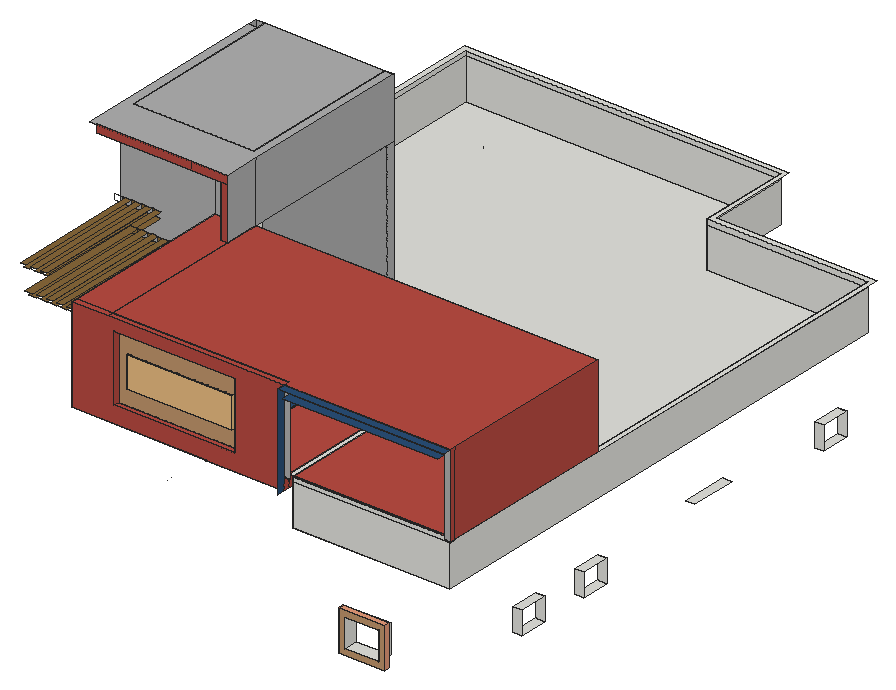
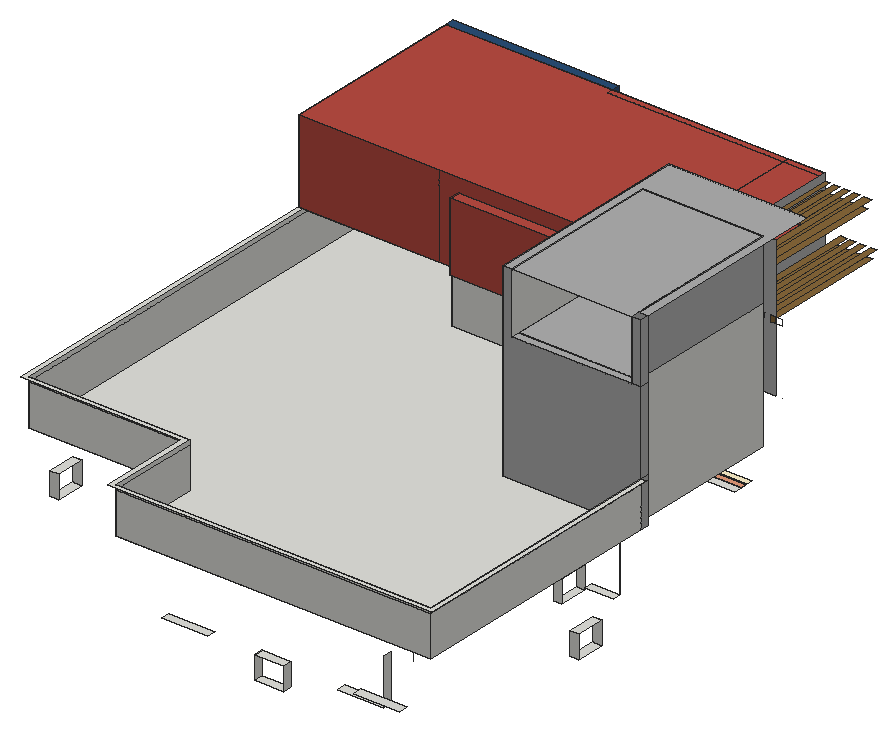
# SketchUp Ruby script. Lengths in inches.
U = 1.inch
M = Sketchup.active_model
def pt(a) = Geom::Point3d.new(a.map { |v| v * U })
def face(e, loops, mat)
  f = e.add_face(loops[0].map { |a| pt(a) })
  loops[1..].each { |l| e.add_face(l.map { |a| pt(a) }).erase! }
  f.material = f.back_material = mat if mat
  f
end
# faces: each face lists its corners as indices into pts; further lists are holes
def faces(e, pts, list, mat = nil) = list.each { |f| face(e, (f[0].is_a?(Array) ? f : [f]).map { |l| l.map { |i| pts[i] } }, mat) }
# xy, xz, yz: faces in a plane at the given z, y or x. An outline is a flat list of corners, or four numbers for a rectangle; further outlines are holes
def ring(l) = l.size == 4 ? [[l[0], l[1]], [l[2], l[1]], [l[2], l[3]], [l[0], l[3]]] : l.each_slice(2).to_a
def flat(e, list, mat, &to3) = list.each { |f| face(e, (f[0].is_a?(Array) ? f : [f]).map { |l| ring(l).map { |u, v| to3.(u, v) } }, mat) }
def xy(e, z, list, mat = nil) = flat(e, list, mat) { |x, y| [x, y, z] }
def xz(e, y, list, mat = nil) = flat(e, list, mat) { |x, z| [x, y, z] }
def yz(e, x, list, mat = nil) = flat(e, list, mat) { |y, z| [x, y, z] }
def lines(e, pts, list) = list.each { |a, b| e.add_line(pt(pts[a]), pt(pts[b])) }
# prism: a flat outline (further loops are holes) pulled along v
def prism(e, loops, v, mat = nil)
  f = face(e, loops, mat); d = Geom::Vector3d.new(v.map { |x| x * U })
  f.pushpull(f.normal.samedirection?(d) ? d.length : -d.length)
end
def box(e, o, s, mat = nil) = prism(e, [[o, [o[0] + s[0], o[1], o[2]], [o[0] + s[0], o[1] + s[1], o[2]], [o[0], o[1] + s[1], o[2]]]], [0, 0, s[2]], mat)
def at(x, y, z, deg = 0) = Geom::Transformation.translation(pt([x, y, z])) * Geom::Transformation.rotation(ORIGIN, Z_AXIS, deg.degrees)
def axes(o, x, y, z) = Geom::Transformation.new([*x, 0, *y, 0, *z, 0, *pt(o).to_a, 1])
def part(name) = M.definitions.add(name)
# library, detail: a bought-in or finely detailed component or shape, given as its bounding box
def library(name, o, s) = part(name).tap { |d| box(d.entities, o, s) }
def detail(e, o, s) = box(e.add_group.entities, o, s)
def put(e, d, t, mat = nil) = e.add_instance(d, t).tap { |i| i.material = mat if mat }
def group(e, t, mat = nil) = e.add_group.tap { |g| g.transformation = t; g.material = mat if mat }.entities
root = M.entities
M.materials.add("Heather_Jeans").color = [86, 117, 147]
M.materials.add("Heather_PantShadow").color = [42, 79, 119]
M.materials.add("Heather_Skin").color = [229, 155, 121]
M.materials.add("K359").color = [135, 104, 58]
M.materials.add("Material~76").color = [176, 176, 176]
M.materials.add("Material~8").color = [65, 47, 38]
M.materials.add("Panel-Opening1").color = [194, 151, 109]
M.materials.add("[Color_D05]").color = [255, 242, 204]
M.materials.add("[Metal Rusted]").color = [184, 75, 66]
M.materials.add("[Polished Concrete New]").color = [200, 200, 203]
c1 = library("Eshavasya",[1,0,0],[56.875,16.44,1])
xy(root,52.62,[[93.01,603.52,141.01,612.52]])
xy(root,54,[[398.62,2.875,446.62,8.875]],"Heather_Skin")
xy(root,60,[[404.62,2.875,440.62,17.875]])
xy(root,66,[[501.9,101.875,510.9,131.875],[501.9,182.875,510.9,212.875],[3.9,439.375,12.9,469.375],[501.9,496.375,510.9,526.375],[158.71,652.375,188.71,661.375]])
xy(root,76.62,[[60.01,390.52,69.01,420.52]])
xy(root,90,[[404.62,2.875,440.62,17.875],[501.9,101.875,510.9,131.875],[395.4,161.875,425.4,167.875],[501.9,182.875,510.9,212.875],[177.5,190.375,249.5,205.375],
  [51.9,196.375,99.9,205.375],[287.9,196.375,327.9,205.375],[501.9,327.95,510.9,375.95],[17.9,397.375,47.9,406.375],[110.9,397.375,150.9,406.375],
  [3.9,439.375,12.9,469.375],[342.9,451.375,399.9,460.375],[399.9,464.375,405.9,494.375],[501.9,496.375,510.9,526.375],[167.9,499.375,203.9,508.375],
  [217.9,499.375,253.9,508.375],[173.9,556.375,203.9,562.375],[36.9,652.375,84.9,661.375],[158.71,652.375,188.71,661.375],[237.9,652.375,285.9,661.375]])
xy(root,90,[[51.9,190.375,99.9,196.375]],"Heather_Skin")
xy(root,96,[[398.62,2.875,446.62,8.875]],"Heather_Skin")
xy(root,96.08,[[45.9,190.375,105.9,196.375]],"[Color_D05]")
xy(root,96.18,[[171.5,190.375,255.5,191.8125]],"Heather_PantShadow")
xy(root,96.18,[[216.0625,191.8125,255.5,196.375]],"[Metal Rusted]")
xy(root,100.62,[[60.01,390.52,69.01,420.52]])
xy(root,108.3125,[[165.5,191.8125,165.55,196.375]],"[Metal Rusted]")
xy(root,108.37,[[165.55,191.8125,171.5,196.375]],"[Metal Rusted]")
xy(root,116.53,[[150.06,191.8125,150.19,196.375]],"[Metal Rusted]")
xy(root,146.6875,[[342.01,13.98,342.01,211.98,153.01,211.98,153.01,381.48,9.01,381.48,9.01,656.27,337.8,656.27,337.8,560.27,505.8,560.27,505.8,13.98],[18.01,210.48,153.01,372.48],[9.01,372.48,144.01,381.48],[144.01,372.48,153.01,381.48]])
xy(root,181.375,[[246.81,8.875,255.5,14.875],[255.5,8.875,336.9,14.875],[150.19,14.875,255.5,191.8125],[255.5,14.875,255.5,191.8125,216.0625,191.8125,216.0625,196.375,336.9,196.375,336.9,14.875]],"[Metal Rusted]")
xy(root,181.78,[[246.81,8.875,255.5,14.875],[150.19,14.875,255.5,186.625]],"Heather_PantShadow")
xy(root,181.78,[[114.62,8.875,246.81,14.875],[114.62,14.875,150.19,196.375],[150.19,186.625,246.81,190.375]],"[Metal Rusted]")
xy(root,189.3,[[153.01,201.48,159.75,211.98],[159.75,201.48,255.5,211.98]])
xy(root,194.6875,[[505.8,13.98,510.9,14.875],[336.9,14.875,342.01,201.48],[505.8,14.875,510.9,201.875],[505.8,201.875,505.8,560.27,337.8,560.27,337.8,656.27,9.01,656.27,9.01,381.48,3.9,381.48,3.9,661.375,342.9,661.375,342.9,565.375,510.9,565.375,510.9,201.875]])
xy(root,194.6875,[[246.81,186.625,255.5,190.375]],"Heather_PantShadow")
xy(root,194.6875,[[342.01,13.98,505.8,14.875],[342.01,14.875,342.01,190.375,363.75,190.375,363.75,201.875,505.8,201.875,505.8,14.875],[342.01,190.375,363.75,201.875],[159.75,196.375,159.75,213.42,342.75,213.42,342.75,211.98,255.5,211.98,255.5,196.375],[255.5,196.375,336.9,201.48],
  [255.5,201.48,336.9,201.875],[336.9,201.48,342.01,201.875],[255.5,201.875,342.01,211.98],[342.01,201.875,342.75,211.98]],"[Metal Rusted]")
xy(root,199.07,[[159.06,8.875,284.74,14.875]],"[Metal Rusted]")
xy(root,256.7,[[21.24,63.6,27.43,196.375],[31.92,63.6,38.11,196.375],[42.76,63.6,48.94,196.375],[52.37,63.6,58.56,196.375]],"K359")
xy(root,262.88,[[21.24,58.375,27.43,196.375],[31.92,58.375,38.11,196.375],[42.76,58.375,48.94,196.375],[52.37,58.375,58.56,196.375]],"K359")
xy(root,266.6875,[[153.01,196.375,159.75,201.875],[159.75,201.875,342.75,213.42]],"[Metal Rusted]")
xy(root,267.3125,[[65.39,14.74,73.21,147.52],[77.35,14.74,83.53,147.52],[88.02,14.74,94.21,147.52],[98.86,14.74,105.05,147.52],[108.47,14.74,114.66,147.52]],"K359")
xy(root,268.82,[[159.06,8.875,284.74,14.875]],"[Metal Rusted]")
xy(root,273.5,[[65.39,9.52,73.21,147.52],[77.35,9.52,83.53,147.52],[88.02,9.52,94.21,147.52],[98.86,9.52,105.05,147.52],[108.47,9.52,114.66,147.52]],"K359")
xy(root,274.0625,[[342.9,0,504.9,8.875]],"Heather_PantShadow")
xy(root,280.625,[[144.01,210.48,153.01,372.48],[9.01,372.48,18.01,381.48],[144.01,372.48,153.01,381.35]])
xy(root,280.625,[[18.01,210.48,144.01,372.48],[18.01,372.48,144.01,381.48]],"Material~76")
xy(root,280.625,[[114.62,8.875,153.01,14.875],[114.62,14.875,114.62,196.375,145.47,196.375,145.47,164.8125,153.01,164.8125,153.01,14.875]],"[Metal Rusted]")
xy(root,280.6875,[[336.9,0,510.9,8.875]],"Heather_PantShadow")
xy(root,280.75,[[153.01,8.875,336.9,14.875],[336.9,8.875,510.9,8.875,510.9,201.875,153.01,201.875,153.01,14.875,336.9,14.875]],"[Metal Rusted]")
xy(root,335.23,[[15.77,164.8125,114.62,196.375],[114.62,164.8125,145.47,196.375]],"[Metal Rusted]")
xy(root,343.875,[[9.01,164.8125,9.01,372.48,18.01,372.48,18.01,210.48,144.01,210.48,144.01,381.35,153.01,381.35,153.01,164.8125],[18.01,210.48,144.01,381.48]],"Material~76")
xz(root,2.875,[[[398.62,54,446.62,96],[404.62,60,440.62,90]]],"Panel-Opening1")
xz(root,8.875,[[336.9,194.1875,342.9,194.6875],[504.9,194.1875,510.9,194.6875]],"Heather_Jeans")
xz(root,8.875,[[336.9,194.6875,342.9,194.6875,342.9,274.0625,504.9,274.0625,504.9,194.6875,510.9,194.6875,510.9,280.6875,336.9,280.6875],[336.9,280.6875,510.9,280.75]],"Material~76")
xz(root,8.875,[[[255.5,181.375,336.9,181.375,336.9,280.75,153.01,280.75,153.01,280.625,114.62,280.625,114.62,181.78,255.5,181.78],[159.06,199.07,284.74,268.82]],[246.81,181.375,255.5,181.375,246.81,181.78],[255.5,181.375,255.5,181.78,246.81,181.78]],"[Metal Rusted]")
xz(root,13.98,[[342.01,146.6875,505.8,189.3],[342.01,189.3,505.8,194.1875]])
xz(root,13.98,[[342.01,194.1875,505.8,194.6875],[505.8,194.1875,510.9,194.6875]],"[Metal Rusted]")
xz(root,14.875,[[246.81,181.375,246.81,181.78,255.5,181.375]])
xz(root,14.875,[[159.06,199.07,284.74,268.82]],"Panel-Opening1")
xz(root,14.875,[[[255.5,181.375,255.5,181.78,150.06,181.78,150.06,280.625,153.01,280.625,153.01,280.75,336.9,280.75,336.9,181.375],[159.06,199.07,284.74,268.82]],[150.19,181.375,246.81,181.78],[255.5,181.375,246.81,181.78,255.5,181.78],[336.9,194.1875,342.01,194.6875]],"[Metal Rusted]")
xz(root,101.875,[[501.9,66,510.9,90]])
xz(root,131.875,[[501.9,66,510.9,90]])
xz(root,147.52,[[73.21,267.3125,77.35,273.5],[83.53,267.3125,88.02,273.5],[94.21,267.3125,98.86,273.5],[105.05,267.3125,108.47,273.5]],"K359")
xz(root,164.8125,[[145.47,280.625,153.01,335.23],[15.77,335.23,114.62,343.875],[114.62,335.23,153.01,343.875]],"[Metal Rusted]")
xz(root,182.875,[[501.9,66,510.9,90]])
xz(root,186.625,[[246.81,181.78,255.5,194.6875]],"Heather_PantShadow")
xz(root,191.8125,[[165.55,108.3125,171.5,108.37]])
xz(root,196.375,[[51.9,89.91,99.9,90]])
xz(root,196.375,[[331.52,181.375,336.9,181.375,336.9,194.6875,255.5,194.6875,255.5,189.3,331.52,189.3]],"Heather_PantShadow")
xz(root,196.375,[[17.11,256.7,21.24,262.88],[27.43,256.7,31.92,262.88],[38.11,256.7,42.76,262.88],[48.94,256.7,52.37,262.88]],"K359")
xz(root,196.375,[[[15.77,189.3,114.62,335.23],[38.11,256.7,42.76,262.88],[27.43,256.7,31.92,262.88],[17.11,256.7,21.24,262.88],[48.94,256.7,52.37,262.88]],[114.62,280.625,145.47,335.23]],"Material~76")
xz(root,196.375,[[114.62,189.3,150.06,194.6875]],"[Metal Rusted]")
xz(root,196.375,[[165.55,96.18,165.55,108.3125,165.5,108.3125],[150.06,116.53,150.19,181.78],[255.5,181.375,331.52,189.3]],"[Polished Concrete New]")
xz(root,201.48,[[150.06,189.3,153.01,194.6875],[153.01,189.3,159.75,194.6875]])
xz(root,201.875,[[342.75,194.6875,342.75,266.6875,153.01,266.6875,153.01,280.75,363.75,280.75,363.75,194.6875],[363.75,194.6875,510.9,280.75]],"[Metal Rusted]")
xz(root,210.48,[[18.01,146.6875,153.01,280.625],[18.01,280.625,144.01,343.875]])
xz(root,211.98,[[153.01,146.6875,342.01,146.6875,342.01,194.6875,255.5,194.6875,255.5,189.3,153.01,189.3]])
xz(root,212.875,[[501.9,66,510.9,90]])
xz(root,213.42,[[159.75,194.6875,342.75,266.6875]],"[Metal Rusted]")
xz(root,372.48,[[9.01,146.6875,18.01,280.625],[18.01,146.6875,153.01,280.625]])
xz(root,381.35,[[144.01,280.625,153.01,343.875]])
xz(root,381.48,[[9.01,146.6875,9.01,280.625,144.01,280.625,144.01,343.875,153.01,343.875,153.01,146.6875],[9.01,280.625,18.01,343.875]],"Material~76")
xz(root,390.52,[[60.01,76.62,69.01,100.62]])
xz(root,420.52,[[60.01,76.62,69.01,100.62]])
xz(root,439.375,[[3.9,66,12.9,90]])
xz(root,460.375,[[342.9,90,399.9,138]])
xz(root,469.375,[[3.9,66,12.9,90]])
xz(root,496.375,[[501.9,66,510.9,90]])
xz(root,526.375,[[501.9,66,510.9,90]])
xz(root,560.27,[[337.8,146.6875,505.8,189.3],[337.8,189.3,505.8,194.6875]])
xz(root,656.27,[[9.01,146.6875,337.8,189.3],[9.01,189.3,337.8,194.6875]])
yz(root,9.01,[[381.48,146.6875,656.27,189.3],[381.48,189.3,656.27,194.6875]])
yz(root,9.01,[[372.48,146.6875,381.48,189.3],[372.48,189.3,381.48,194.6875],[372.48,194.6875,381.48,280.625],[372.48,280.625,381.48,343.875]],"Material~76")
yz(root,17.9,[[397.375,90,397.41,138]])
yz(root,18.01,[[210.48,146.6875,372.48,280.625]])
yz(root,18.01,[[210.48,280.625,381.48,343.875]],"Material~76")
yz(root,51.9,[[190.375,89.91,196.375,90]],"Heather_Skin")
yz(root,93.01,[[603.52,52.62,612.52,100.62]])
yz(root,99.9,[[190.375,89.91,196.375,90]],"Heather_Skin")
yz(root,114.62,[[8.875,194.6875,196.375,280.625]],"Material~76")
yz(root,114.62,[[8.875,181.78,196.375,194.6875]],"[Metal Rusted]")
yz(root,144.01,[[210.48,280.625,381.35,343.875],[381.35,280.625,381.48,343.875]])
yz(root,145.47,[[164.8125,280.625,196.375,335.23]],"[Metal Rusted]")
yz(root,150.06,[[196.375,189.3,201.48,194.6875]])
yz(root,150.19,[[191.8125,116.53,191.8125,181.375,14.875,181.375,14.875,181.78,196.375,181.78,196.375,116.53]],"[Metal Rusted]")
yz(root,153.01,[[201.48,146.6875,210.48,189.3],[210.48,146.6875,211.98,189.3]])
yz(root,153.01,[[211.98,146.6875,372.48,146.6875,372.48,280.625,210.48,280.625,210.48,189.3,211.98,189.3],[372.48,146.6875,381.48,280.625],[201.875,280.625,201.875,280.75,201.48,280.75,201.48,343.875,381.35,343.875,381.35,280.625],[164.8125,280.75,201.48,343.875]],"Material~76")
yz(root,153.01,[[196.375,266.6875,196.375,280.625,164.8125,280.625,164.8125,280.75,201.875,280.75,201.875,266.6875],[8.875,280.625,14.875,280.75],[14.875,280.625,164.8125,280.75]],"[Metal Rusted]")
yz(root,158.71,[[652.375,66,661.375,90]])
yz(root,159.06,[[8.875,199.07,14.875,268.82]],"[Metal Rusted]")
yz(root,159.75,[[196.375,194.6875,213.42,266.6875]],"[Metal Rusted]")
yz(root,165.55,[[190.375,96.18,196.375,108.3125],[191.8125,108.3125,196.375,108.37]],"[Metal Rusted]")
yz(root,188.71,[[652.375,66,661.375,90]])
yz(root,216.0625,[[191.8125,96.18,196.375,181.375]],"[Metal Rusted]")
yz(root,246.81,[[186.625,181.78,190.375,194.6875]],"Heather_PantShadow")
yz(root,246.81,[[8.875,181.375,14.875,181.78]],"[Metal Rusted]")
yz(root,255.5,[[201.48,189.3,211.98,194.6875]])
yz(root,255.5,[[186.625,181.78,190.375,194.6875]],"Heather_PantShadow")
yz(root,255.5,[[8.875,181.375,14.875,181.78],[14.875,181.375,190.375,181.78]],"[Metal Rusted]")
yz(root,284.74,[[8.875,199.07,14.875,268.82]],"[Metal Rusted]")
yz(root,336.9,[[0,181.375,8.875,280.6875]],"Heather_PantShadow")
yz(root,336.9,[[8.875,181.375,14.875,194.1875],[14.875,181.375,196.375,194.6875]],"[Metal Rusted]")
yz(root,336.9,[[8.875,194.1875,14.875,194.6875]],"[Polished Concrete New]")
yz(root,337.8,[[560.27,146.6875,656.27,189.3],[560.27,189.3,656.27,194.6875]])
yz(root,342.01,[[13.98,146.6875,13.98,189.3,201.48,189.3,201.48,194.6875,211.98,194.6875,211.98,146.6875],[13.98,189.3,13.98,194.1875,14.875,194.1875,14.875,194.6875,201.48,194.6875,201.48,189.3],[13.98,194.1875,14.875,194.6875]])
yz(root,342.75,[[201.875,194.6875,213.42,266.6875]],"[Metal Rusted]")
yz(root,398.62,[[2.875,54,8.875,90],[2.875,90,8.875,96]],"Heather_Skin")
yz(root,404.62,[[2.875,60,17.875,90]])
yz(root,440.62,[[2.875,60,17.875,90]])
yz(root,446.62,[[2.875,54,8.875,96]],"Heather_Skin")
yz(root,505.8,[[13.98,146.6875,560.27,189.3],[13.98,189.3,560.27,194.6875]])
yz(root,510.9,[[8.875,194.1875,13.98,194.6875],[8.875,194.6875,14.875,280.75],[14.875,194.6875,201.875,280.75]],"[Metal Rusted]")
p = [[165.55,191.8125,96.18],[165.55,190.375,96.18],[171.25,190.375,96.2],[171.25,191.8125,96.2],[165.5,196.375,108.3125],[165.5,191.8125,108.3125],
  [165.55,196.375,96.18],[171.25,196.375,96.2],[246.81,14.875,181.78],[255.5,14.875,181.375],[255.5,8.875,181.375],[246.81,8.875,181.78],
  [9.29,196.375,262.88],[15.77,196.375,262.88],[9.29,196.375,256.7],[17.11,196.375,256.7],[15.77,196.375,256.7],[27.43,63.6,256.7],
  [31.92,63.6,256.7],[38.11,63.6,256.7],[42.76,63.6,256.7],[48.94,63.6,256.7],[52.37,63.6,256.7],[153.01,201.48,194.6875],
  [153.01,190.375,194.6875],[159.75,196.375,194.6875],[159.75,190.375,194.6875],[69.01,603.52,100.62],[69.01,603.52,148.62],[108.01,147.52,52.62],
  [108.04,147.52,52.62],[65.11,332.62,157.3],[65.11,332.62,205.3],[94.21,14.74,267.3125],[98.86,14.74,267.3125],[73.21,14.74,267.3125],
  [77.35,14.74,267.3125],[83.53,14.74,267.3125],[88.02,14.74,267.3125],[105.05,14.74,267.3125],[108.47,14.74,267.3125],[108.01,141.52,52.62],
  [108.04,141.52,52.62],[108.04,147.52,100.52],[108.01,147.52,100.52],[65.11,147.52,199.92],[65.39,147.52,199.92],[150.06,14.875,194.6875],
  [114.62,14.875,194.6875],[9.01,196.375,189.3],[9.29,196.375,189.3],[17.11,196.375,262.88],[153.01,381.48,343.875],[153.01,381.35,343.875],
  [246.81,186.625,194.6875],[246.81,14.875,194.6875],[255.5,186.625,194.6875],[255.5,14.875,194.6875]]
faces(root,p,[[0,1,2,3]])
faces(root,p,[[4,5,0,6],[6,0,3,7],[8,9,10,11]],"[Metal Rusted]")
lines(root,p,[[12,13],[14,12],[15,16],[17,18],[19,20],[21,22],[23,24],[25,26],[27,28],[29,30],[31,32],[33,34],
  [35,36],[37,38],[39,40],[41,42],[43,44],[45,46],[47,48],[49,50],[13,51],[16,14],[52,53],[54,55],
  [56,57]])
put(root,c1,axes([166.86,14.875,216.1],[1.935,0,0],[0,0,1.935],[0,-1.935,0]),"Material~8")
